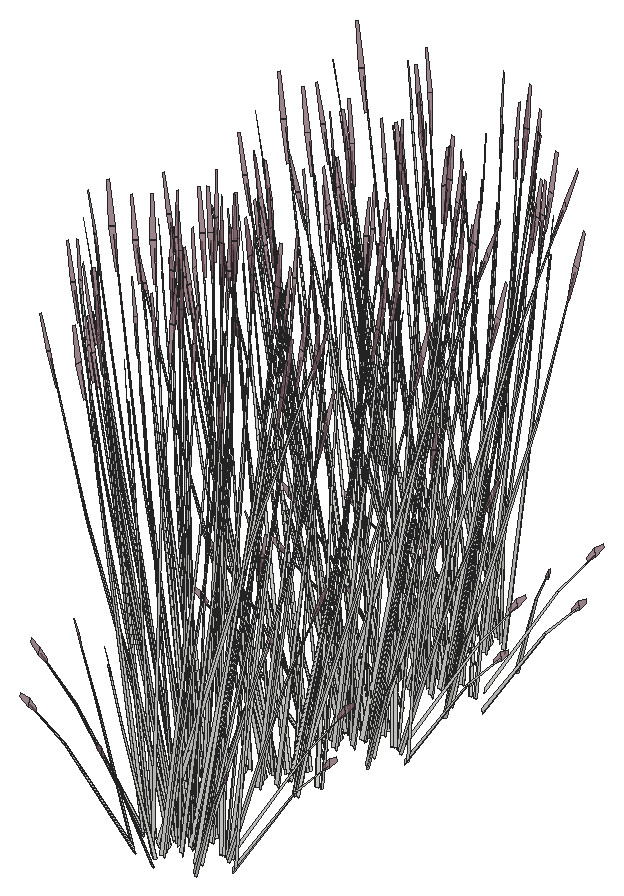
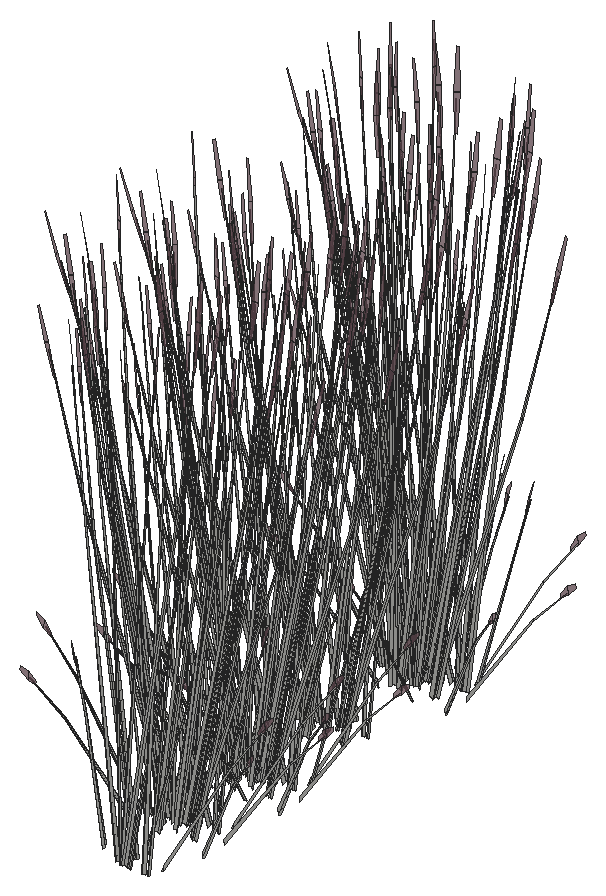
# SketchUp Ruby script. Lengths in inches.
U = 1.inch
M = Sketchup.active_model
def pt(a) = Geom::Point3d.new(a.map { |v| v * U })
def face(e, loops, mat)
  f = e.add_face(loops[0].map { |a| pt(a) })
  loops[1..].each { |l| e.add_face(l.map { |a| pt(a) }).erase! }
  f.material = f.back_material = mat if mat
  f
end
# faces: each face lists its corners as indices into pts; further lists are holes
def faces(e, pts, list, mat = nil) = list.each { |f| face(e, (f[0].is_a?(Array) ? f : [f]).map { |l| l.map { |i| pts[i] } }, mat) }
# xy, xz, yz: faces in a plane at the given z, y or x. An outline is a flat list of corners, or four numbers for a rectangle; further outlines are holes
def ring(l) = l.size == 4 ? [[l[0], l[1]], [l[2], l[1]], [l[2], l[3]], [l[0], l[3]]] : l.each_slice(2).to_a
def flat(e, list, mat, &to3) = list.each { |f| face(e, (f[0].is_a?(Array) ? f : [f]).map { |l| ring(l).map { |u, v| to3.(u, v) } }, mat) }
def xy(e, z, list, mat = nil) = flat(e, list, mat) { |x, y| [x, y, z] }
def xz(e, y, list, mat = nil) = flat(e, list, mat) { |x, z| [x, y, z] }
def yz(e, x, list, mat = nil) = flat(e, list, mat) { |y, z| [x, y, z] }
def lines(e, pts, list) = list.each { |a, b| e.add_line(pt(pts[a]), pt(pts[b])) }
# prism: a flat outline (further loops are holes) pulled along v
def prism(e, loops, v, mat = nil)
  f = face(e, loops, mat); d = Geom::Vector3d.new(v.map { |x| x * U })
  f.pushpull(f.normal.samedirection?(d) ? d.length : -d.length)
end
def box(e, o, s, mat = nil) = prism(e, [[o, [o[0] + s[0], o[1], o[2]], [o[0] + s[0], o[1] + s[1], o[2]], [o[0], o[1] + s[1], o[2]]]], [0, 0, s[2]], mat)
def at(x, y, z, deg = 0) = Geom::Transformation.translation(pt([x, y, z])) * Geom::Transformation.rotation(ORIGIN, Z_AXIS, deg.degrees)
def axes(o, x, y, z) = Geom::Transformation.new([*x, 0, *y, 0, *z, 0, *pt(o).to_a, 1])
def part(name) = M.definitions.add(name)
# library, detail: a bought-in or finely detailed component or shape, given as its bounding box
def library(name, o, s) = part(name).tap { |d| box(d.entities, o, s) }
def detail(e, o, s) = box(e.add_group.entities, o, s)
def put(e, d, t, mat = nil) = e.add_instance(d, t).tap { |i| i.material = mat if mat }
def group(e, t, mat = nil) = e.add_group.tap { |g| g.transformation = t; g.material = mat if mat }.entities
root = M.entities
M.materials.add("LightPink_Translucent").color = [144, 107, 117]
M.materials["LightPink_Translucent"].alpha = 0.75
c1 = part("blade")
p = [[2.15,0.21,22],[0,0.17,0],[0.09,0.45,0],[2.18,0.31,22],[2.29,0.31,22],[0.38,0.45,0],
  [2.48,0.24,33],[2.49,0.24,33],[2.48,0.22,33]]
faces(c1.entities,p,[[0,1,2,3],[4,5,2,3],[6,3,4,7],[8,0,3,6]])
c2 = part("seeds")
p = [[0.3,-0.1,1.38],[-0.01,-0.03,1.59],[-0.01,-0.03,0.03],[0.14,-0.07,-0.07],[0.29,-0.03,3],[0.15,0.01,3.11]]
faces(c2.entities,p,[[0,1,2,3],[1,0,4,5]],"LightPink_Translucent")
c3 = part("blade with seeds")
put(c3.entities,c1,at(0,0,0))
put(c3.entities,c2,axes([2.4,0.25,30.99],[1.5799,-0.05474,1.17369],[-0.12525,1.92788,0.29478],[-0.07173,-0.02425,1.56792]))
put(root,c3,axes([272.2,320.66,123.6],[-0.15005,0.02351,1.76342],[-0.82981,-0.26461,-0.26939],[0.01392,-0.22072,0.30037]))
put(root,c3,axes([269.52,321.47,123.6],[-0.08666,0.08595,1.76342],[-0.87574,0.18531,-0.26939],[-0.21156,-0.16858,0.30037]))
put(root,c3,axes([270.97,323.83,124.2],[-0.36739,-0.66907,-0.69835],[1.05831,-0.24096,-0.18329],[-0.04061,-0.22656,1.54149]))
put(root,c3,axes([275.88,321.79,123.6],[-0.1339,-0.0514,1.76342],[-0.34394,-0.57425,-0.26939],[0.23202,-0.15583,0.30037]))
put(root,c3,axes([270.82,321.91,124.48],[-0.55932,-0.6538,0],[0.93577,-0.36461,-0.51607],[0.21313,-0.08304,1.63711]))
put(root,c3,axes([272.05,321.12,124.23],[-0.61821,0.37431,-0.03893],[-0.56645,-0.40995,-0.17649],[-0.03988,-0.11616,0.58215]))
put(root,c3,axes([268.8,323.74,124.125],[0,-0.65246,-0.49651],[1.00089,0,0],[0,-0.1486,1.57504]))
put(root,c3,axes([271.58,321.81,124.125],[0.83726,-0.32623,-0.49651],[0.50045,0.58498,0],[0.19069,-0.0743,1.57504]))
put(root,c3,axes([272.57,323.15,124.17],[0.60257,-0.49041,-0.62353],[0.74854,0.44469,-0.16365],[0.24146,-0.12234,1.37633]))
put(root,c3,axes([271.53,324.01,124.32],[0.43405,-0.58792,-0.44739],[0.90188,0.28295,0.21531],[0,-0.13553,1.43643]))
put(root,c3,axes([271.92,323.72,124.77],[-0.10425,-0.7445,-0.29095],[1.08575,-0.04502,-0.50002],[0.19119,-0.09917,1.59708]))
put(root,c3,axes([269.23,323.75,124.14],[0.62448,-0.40708,-0.30978],[0.62448,0.40708,0.30978],[0,-0.13112,1.38974]))
put(root,c3,axes([268.98,321.8,124.23],[-0.25807,0.53277,-0.03893],[-0.79428,-0.16389,-0.17649],[-0.1206,-0.08714,0.58215]))
put(root,c3,axes([271.42,324.5,124.77],[-1.00749,-0.31132,-0.29095],[0.48511,-0.65709,-0.50002],[-0.03166,-0.16133,1.59708]))
put(root,c3,axes([268.55,324.23,124.48],[-1.11865,0,0],[0,-0.72922,-0.51607],[0,-0.16609,1.63711]))
put(root,c3,axes([271.78,322.07,124.14],[0.83462,0.16144,-0.30978],[-0.21015,0.56852,0.30978],[0.16826,-0.06556,1.38974]))
put(root,c3,axes([269.42,324.04,124.4375],[-0.83213,0.54855,0.30756],[-0.83263,-0.54278,-0.36492],[-0.02906,-0.15578,1.64885]))
put(root,c3,axes([271.67,325.1875,124.55],[0.23711,-0.77313,-0.23429],[1.12425,0.13477,0.51271],[-0.19645,-0.10677,1.5644]))
put(root,c3,axes([274.94,322.07,124.48],[0.55932,-0.6538,0],[0.93577,0.36461,-0.51607],[0.21313,0.08304,1.63711]))
put(root,c3,axes([271.59,324.87,124.32],[-0.53742,-0.54764,-0.44739],[0.81403,-0.38564,0.21531],[-0.17391,-0.06776,1.43643]))
put(root,c3,axes([277.14,324.66,124.09],[-0.57619,0.0783,1.41583],[-0.09171,-0.62326,0.08104],[0.40356,-0.09434,0.80566]))
put(root,c3,axes([278.19,324.11,124.37],[-0.55463,-0.41721,-0.06488],[0.60744,-0.38228,-0.29416],[0.17212,-0.02691,0.97024]))
put(root,c3,axes([273.1,324.16,124.3125],[0,-0.75495,0],[1.11865,0,0],[0,0,1.79456]))
put(root,c3,axes([271.11,325.08,124.17],[-0.9306,-0.10697,-0.62353],[0.19638,-0.65984,-0.16365],[-0.27771,-0.07995,1.37633]))
put(root,c3,axes([273.38,324.75,124.4],[-0.83213,-0.56158,-0.06131],[0.83263,-0.56193,0],[-0.02906,-0.01961,1.75571]))
put(root,c3,axes([270.89,323.23,123.7],[-0.88056,0.26122,1.28929],[-0.28027,-0.74951,0.50096],[0.54072,0.01247,1.46642]))
put(root,c3,axes([277.77,324.25,123.6],[-0.04675,-0.09906,1.76342],[0.32428,-0.57943,-0.26939],[0.32711,-0.00833,0.30037]))
put(root,c3,axes([268.12,324.15,123.6],[0.02269,0.10283,1.76342],[-0.45738,0.53699,-0.26939],[-0.32488,-0.02707,0.30037]))
put(root,c3,axes([270.12,326.09,124.14],[-0.21015,-0.56852,-0.30978],[0.83462,-0.16144,0.30978],[-0.16826,-0.06556,1.38974]))
put(root,c3,axes([273.17,323.62,124.77],[0.90324,-0.43318,-0.29095],[0.60064,0.61207,-0.50002],[0.22285,0.06216,1.59708]))
put(root,c3,axes([269.89,326.33,124.125],[-0.83726,-0.32623,-0.49651],[0.50045,-0.58498,0],[-0.19069,-0.0743,1.57504]))
put(root,c3,axes([275.45,322.47,124.125],[0.83726,0.32623,-0.49651],[-0.50045,0.58498,0],[0.19069,0.0743,1.57504]))
put(root,c3,axes([273.86,324.33,124.3125],[1.00089,0,0],[0,0.67548,0],[0,0,1.78407]))
put(root,c3,axes([272.17,325.18,124.77],[-0.90324,0.43318,-0.29095],[-0.60064,-0.61207,-0.50002],[-0.22285,-0.06216,1.59708]))
put(root,c3,axes([275.22,322.71,124.14],[0.21015,0.56852,-0.30978],[-0.83462,0.16144,0.30978],[0.16826,0.06556,1.38974]))
put(root,c3,axes([272.64,325.9,124.3125],[-0.29189,-0.56252,0],[0.83351,-0.19699,0],[0,0,1.54371]))
put(root,c3,axes([273.73,325.82,124.29],[0.93921,-0.22138,-0.19198],[0.33003,0.6377,0.00008],[0.10367,-0.02447,1.73897]))
put(root,c3,axes([273.84,324.62,124.32],[0.62448,0.42144,0],[-0.62448,0.42144,0],[0,0,1.69266]))
put(root,c3,axes([274.23,323.72,124.17],[0.9306,0.10697,-0.62353],[-0.19638,0.65984,-0.16365],[0.27771,0.07995,1.37633]))
put(root,c3,axes([272.43,326.16,124.3],[-0.90188,-0.29293,0],[0.43405,-0.60866,0],[0,0,1.62707]))
put(root,c3,axes([273.18,325.38,124.57],[-0.87356,-0.52515,-0.25192],[0.73507,-0.5897,0.5513],[-0.23523,0.06143,1.68216]))
put(root,c3,axes([273.67,324.46,124.4],[0,0.75458,-0.05637],[-1.11865,0,0],[0,0.02371,1.79368]))
put(root,c3,axes([273.75,323.93,124.32],[0.53742,0.54764,-0.44739],[-0.81403,0.38564,0.21531],[0.17391,0.06776,1.43643]))
put(root,c3,axes([270.4,326.72,124.48],[-0.55932,0.6538,0],[-0.93577,-0.36461,-0.51607],[-0.21313,-0.08304,1.63711]))
put(root,c3,axes([272.74,325.27,124.32],[-0.97146,0.04028,-0.44739],[-0.08785,-0.66859,0.21531],[-0.17391,0.06776,1.43643]))
put(root,c3,axes([273.45,326.17,124.3125],[0.90188,0.29293,0],[-0.43405,0.60866,0],[0,0,1.74954]))
put(root,c3,axes([273.8125,326.82,124.3],[-0.55235,-0.65609,-0.05142],[0.93577,-0.36461,0.51607],[-0.23059,0.06247,1.6363]))
put(root,c3,axes([273.13,325.92,124.4],[0.38895,0.74956,-0.06012],[-1.11135,0.26265,0],[0.01358,0.02618,1.72173]))
put(root,c3,axes([273.5625,326.73,124.14],[-0.83462,-0.16144,-0.30978],[0.21015,-0.56852,0.30978],[-0.16826,0.06556,1.38974]))
put(root,c3,axes([276.79,324.56,124.48],[1.11865,0,0],[0,0.72922,-0.51607],[0,0.16609,1.63711]))
put(root,c3,axes([276.34,324.9375,124.31],[-1.1181,-0.00522,-0.04976],[0,-0.72922,0.49943],[-0.03514,0.166,1.58352]))
put(root,c3,axes([273.92,324.3,124.77],[1.00749,0.31132,-0.29095],[-0.48511,0.65709,-0.50002],[0.03166,0.16133,1.59708]))
put(root,c3,axes([276.11,325.05,124.14],[-0.62448,0.40708,-0.30978],[-0.62448,-0.40708,0.30978],[0,0.13112,1.38974]))
put(root,c3,axes([273.42,325.08,124.77],[0.10425,0.7445,-0.29095],[-1.08575,0.04502,-0.50002],[-0.19119,0.09917,1.59708]))
put(root,c3,axes([273.81,324.79,124.32],[-0.43405,0.58792,-0.44739],[-0.90188,-0.28295,0.21531],[0,0.13553,1.43643]))
put(root,c3,axes([272.77,325.65,124.17],[-0.60257,0.49041,-0.62353],[-0.74854,-0.44469,-0.16365],[-0.24146,0.12234,1.37633]))
put(root,c3,axes([273.84,326.48,124.4375],[1.11998,0.21207,0.30756],[-0.2802,0.75803,-0.36492],[-0.18537,0.09487,1.64885]))
put(root,c3,axes([273.76,326.99,124.125],[-0.83726,0.32623,-0.49651],[-0.50045,-0.58498,0],[-0.19069,0.0743,1.57504]))
put(root,c3,axes([276.54,325.06,124.125],[0,0.65246,-0.49651],[-1.00089,0,0],[0,0.1486,1.57504]))
put(root,c3,axes([274.52,326.89,124.48],[0.55932,0.6538,0],[-0.93577,0.36461,-0.51607],[-0.21313,0.08304,1.63711]))
put(root,c3,axes([275.41,327.11,123.6],[0.06518,-0.0942,1.76342],[0.82057,-0.27742,-0.26939],[0.24877,0.14358,0.30037]))
put(root,c3,axes([274.33,324.97,124.2],[0.32803,0.59738,-0.69212],[-0.94492,0.21515,-0.18165],[0.03626,0.20229,1.52773]))
put(root,c3,axes([267.875,327.03,123.6],[0.12,0.06519,1.76342],[0.20347,0.60397,-0.26939],[-0.26596,0.12879,0.30037]))
put(root,c3,axes([271.58,327.09,123.6],[0.14478,-0.0355,1.76342],[0.8709,0.19542,-0.26939],[0.02547,0.22025,0.30037]))
put(root,c3,axes([270.97,336.8125,125.11],[-0.36739,-0.66907,-0.69835],[1.05831,-0.24096,-0.18329],[-0.04061,-0.22656,1.54149]))
put(root,c3,axes([268.8,336.72,125.03],[0,-0.65246,-0.49651],[1.00089,0,0],[0,-0.1486,1.57504]))
put(root,c3,axes([271.58,334.79,125.03],[0.83726,-0.32623,-0.49651],[0.50045,0.58498,0],[0.19069,-0.0743,1.57504]))
put(root,c3,axes([272.57,336.125,125.07],[0.60257,-0.49041,-0.62353],[0.74854,0.44469,-0.16365],[0.24146,-0.12234,1.37633]))
put(root,c3,axes([271.53,336.98,125.22],[0.43405,-0.58792,-0.44739],[0.90188,0.28295,0.21531],[0,-0.13553,1.43643]))
put(root,c3,axes([269.23,336.73,125.04],[0.62448,-0.40708,-0.30978],[0.62448,0.40708,0.30978],[0,-0.13112,1.38974]))
put(root,c3,axes([271.78,335.04,125.04],[0.83462,0.16144,-0.30978],[-0.21015,0.56852,0.30978],[0.16826,-0.06556,1.38974]))
put(root,c3,axes([271.59,337.85,125.22],[-0.53742,-0.54764,-0.44739],[0.81403,-0.38564,0.21531],[-0.17391,-0.06776,1.43643]))
put(root,c3,axes([271.11,338.06,125.07],[-0.9306,-0.10697,-0.62353],[0.19638,-0.65984,-0.16365],[-0.27771,-0.07995,1.37633]))
put(root,c3,axes([270.12,339.06,125.04],[-0.21015,-0.56852,-0.30978],[0.83462,-0.16144,0.30978],[-0.16826,-0.06556,1.38974]))
put(root,c3,axes([269.89,339.31,125.03],[-0.83726,-0.32623,-0.49651],[0.50045,-0.58498,0],[-0.19069,-0.0743,1.57504]))
put(root,c3,axes([275.45,335.45,125.03],[0.83726,0.32623,-0.49651],[-0.50045,0.58498,0],[0.19069,0.0743,1.57504]))
put(root,c3,axes([275.22,335.6875,125.04],[0.21015,0.56852,-0.30978],[-0.83462,0.16144,0.30978],[0.16826,0.06556,1.38974]))
put(root,c3,axes([274.23,336.69,125.07],[0.9306,0.10697,-0.62353],[-0.19638,0.65984,-0.16365],[0.27771,0.07995,1.37633]))
put(root,c3,axes([273.75,336.9,125.22],[0.53742,0.54764,-0.44739],[-0.81403,0.38564,0.21531],[0.17391,0.06776,1.43643]))
put(root,c3,axes([272.74,338.24,125.22],[-0.97146,0.04028,-0.44739],[-0.08785,-0.66859,0.21531],[-0.17391,0.06776,1.43643]))
put(root,c3,axes([272.2,343.92,123.82],[-0.15005,0.02351,1.76342],[-0.82981,-0.26461,-0.26939],[0.01392,-0.22072,0.30037]))
put(root,c3,axes([273.5625,339.71,125.04],[-0.83462,-0.16144,-0.30978],[0.21015,-0.56852,0.30978],[-0.16826,0.06556,1.38974]))
put(root,c3,axes([276.11,338.02,125.04],[-0.62448,0.40708,-0.30978],[-0.62448,-0.40708,0.30978],[0,0.13112,1.38974]))
put(root,c3,axes([273.81,337.77,125.22],[-0.43405,0.58792,-0.44739],[-0.90188,-0.28295,0.21531],[0,0.13553,1.43643]))
put(root,c3,axes([272.77,338.63,125.07],[-0.60257,0.49041,-0.62353],[-0.74854,-0.44469,-0.16365],[-0.24146,0.12234,1.37633]))
put(root,c3,axes([273.76,339.97,125.03],[-0.83726,0.32623,-0.49651],[-0.50045,-0.58498,0],[-0.19069,0.0743,1.57504]))
put(root,c3,axes([276.54,338.04,125.03],[0,0.65246,-0.49651],[-1.00089,0,0],[0,0.1486,1.57504]))
put(root,c3,axes([269.52,344.72,123.82],[-0.08666,0.08595,1.76342],[-0.87574,0.18531,-0.26939],[-0.21156,-0.16858,0.30037]))
put(root,c3,axes([270.97,347.09,124.42],[-0.36739,-0.66907,-0.69835],[1.05831,-0.24096,-0.18329],[-0.04061,-0.22656,1.54149]))
put(root,c3,axes([275.88,345.04,123.82],[-0.1339,-0.0514,1.76342],[-0.34394,-0.57425,-0.26939],[0.23202,-0.15583,0.30037]))
put(root,c3,axes([274.33,337.95,125.11],[0.32803,0.59738,-0.69212],[-0.94492,0.21515,-0.18165],[0.03626,0.20229,1.52773]))
put(root,c3,axes([272.05,344.375,124.45],[-0.61821,0.37431,-0.03893],[-0.56645,-0.40995,-0.17649],[-0.03988,-0.11616,0.58215]))
put(root,c3,axes([268.8,346.99,124.34],[0,-0.65246,-0.49651],[1.00089,0,0],[0,-0.1486,1.57504]))
put(root,c3,axes([271.58,345.0625,124.34],[0.83726,-0.32623,-0.49651],[0.50045,0.58498,0],[0.19069,-0.0743,1.57504]))
put(root,c3,axes([272.57,346.4,124.38],[0.60257,-0.49041,-0.62353],[0.74854,0.44469,-0.16365],[0.24146,-0.12234,1.37633]))
put(root,c3,axes([271.53,347.26,124.53],[0.43405,-0.58792,-0.44739],[0.90188,0.28295,0.21531],[0,-0.13553,1.43643]))
put(root,c3,axes([271.92,346.97,124.99],[-0.10425,-0.7445,-0.29095],[1.08575,-0.04502,-0.50002],[0.19119,-0.09917,1.59708]))
put(root,c3,axes([269.23,347.01,124.35],[0.62448,-0.40708,-0.30978],[0.62448,0.40708,0.30978],[0,-0.13112,1.38974]))
put(root,c3,axes([268.98,345.06,124.45],[-0.25807,0.53277,-0.03893],[-0.79428,-0.16389,-0.17649],[-0.1206,-0.08714,0.58215]))
put(root,c3,axes([271.42,347.75,124.99],[-1.00749,-0.31132,-0.29095],[0.48511,-0.65709,-0.50002],[-0.03166,-0.16133,1.59708]))
put(root,c3,axes([271.78,345.32,124.35],[0.83462,0.16144,-0.30978],[-0.21015,0.56852,0.30978],[0.16826,-0.06556,1.38974]))
put(root,c3,axes([271.67,348.4375,124.76],[0.23711,-0.77313,-0.23429],[1.12425,0.13477,0.51271],[-0.19645,-0.10677,1.5644]))
put(root,c3,axes([271.59,348.125,124.53],[-0.53742,-0.54764,-0.44739],[0.81403,-0.38564,0.21531],[-0.17391,-0.06776,1.43643]))
put(root,c3,axes([277.14,347.91,124.31],[-0.57619,0.0783,1.41583],[-0.09171,-0.62326,0.08104],[0.40356,-0.09434,0.80566]))
put(root,c3,axes([278.19,347.36,124.58],[-0.55463,-0.41721,-0.06488],[0.60744,-0.38228,-0.29416],[0.17212,-0.02691,0.97024]))
put(root,c3,axes([271.11,348.33,124.38],[-0.9306,-0.10697,-0.62353],[0.19638,-0.65984,-0.16365],[-0.27771,-0.07995,1.37633]))
put(root,c3,axes([270.89,346.49,123.92],[-0.88056,0.26122,1.28929],[-0.28027,-0.74951,0.50096],[0.54072,0.01247,1.46642]))
put(root,c3,axes([277.77,347.5,123.82],[-0.04675,-0.09906,1.76342],[0.32428,-0.57943,-0.26939],[0.32711,-0.00833,0.30037]))
put(root,c3,axes([268.12,347.4,123.82],[0.02269,0.10283,1.76342],[-0.45738,0.53699,-0.26939],[-0.32488,-0.02707,0.30037]))
put(root,c3,axes([270.12,349.34,124.35],[-0.21015,-0.56852,-0.30978],[0.83462,-0.16144,0.30978],[-0.16826,-0.06556,1.38974]))
put(root,c3,axes([273.17,346.87,124.99],[0.90324,-0.43318,-0.29095],[0.60064,0.61207,-0.50002],[0.22285,0.06216,1.59708]))
put(root,c3,axes([269.89,349.58,124.34],[-0.83726,-0.32623,-0.49651],[0.50045,-0.58498,0],[-0.19069,-0.0743,1.57504]))
put(root,c3,axes([275.45,345.72,124.34],[0.83726,0.32623,-0.49651],[-0.50045,0.58498,0],[0.19069,0.0743,1.57504]))
put(root,c3,axes([272.17,348.43,124.99],[-0.90324,0.43318,-0.29095],[-0.60064,-0.61207,-0.50002],[-0.22285,-0.06216,1.59708]))
put(root,c3,axes([275.22,345.96,124.35],[0.21015,0.56852,-0.30978],[-0.83462,0.16144,0.30978],[0.16826,0.06556,1.38974]))
put(root,c3,axes([273.73,349.08,124.51],[0.93921,-0.22138,-0.19198],[0.33003,0.6377,0.00008],[0.10367,-0.02447,1.73897]))
put(root,c3,axes([274.23,346.97,124.38],[0.9306,0.10697,-0.62353],[-0.19638,0.65984,-0.16365],[0.27771,0.07995,1.37633]))
put(root,c3,axes([273.18,348.63,124.79],[-0.87356,-0.52515,-0.25192],[0.73507,-0.5897,0.5513],[-0.23523,0.06143,1.68216]))
put(root,c3,axes([273.75,347.18,124.53],[0.53742,0.54764,-0.44739],[-0.81403,0.38564,0.21531],[0.17391,0.06776,1.43643]))
put(root,c3,axes([272.74,348.52,124.53],[-0.97146,0.04028,-0.44739],[-0.08785,-0.66859,0.21531],[-0.17391,0.06776,1.43643]))
put(root,c3,axes([273.8125,350.07,124.52],[-0.55235,-0.65609,-0.05142],[0.93577,-0.36461,0.51607],[-0.23059,0.06247,1.6363]))
put(root,c3,axes([272.2,354.45,124.14],[-0.15005,0.02351,1.76342],[-0.82981,-0.26461,-0.26939],[0.01392,-0.22072,0.30037]))
put(root,c3,axes([273.5625,349.99,124.35],[-0.83462,-0.16144,-0.30978],[0.21015,-0.56852,0.30978],[-0.16826,0.06556,1.38974]))
put(root,c3,axes([276.34,348.19,124.52],[-1.1181,-0.00522,-0.04976],[0,-0.72922,0.49943],[-0.03514,0.166,1.58352]))
put(root,c3,axes([273.92,347.56,124.99],[1.00749,0.31132,-0.29095],[-0.48511,0.65709,-0.50002],[0.03166,0.16133,1.59708]))
put(root,c3,axes([276.11,348.3,124.35],[-0.62448,0.40708,-0.30978],[-0.62448,-0.40708,0.30978],[0,0.13112,1.38974]))
put(root,c3,axes([273.42,348.34,124.99],[0.10425,0.7445,-0.29095],[-1.08575,0.04502,-0.50002],[-0.19119,0.09917,1.59708]))
put(root,c3,axes([273.81,348.05,124.53],[-0.43405,0.58792,-0.44739],[-0.90188,-0.28295,0.21531],[0,0.13553,1.43643]))
put(root,c3,axes([272.77,348.91,124.38],[-0.60257,0.49041,-0.62353],[-0.74854,-0.44469,-0.16365],[-0.24146,0.12234,1.37633]))
put(root,c3,axes([273.76,350.24,124.34],[-0.83726,0.32623,-0.49651],[-0.50045,-0.58498,0],[-0.19069,0.0743,1.57504]))
put(root,c3,axes([276.54,348.3125,124.34],[0,0.65246,-0.49651],[-1.00089,0,0],[0,0.1486,1.57504]))
put(root,c3,axes([269.52,355.26,124.14],[-0.08666,0.08595,1.76342],[-0.87574,0.18531,-0.26939],[-0.21156,-0.16858,0.30037]))
put(root,c3,axes([270.97,357.62,124.74],[-0.36739,-0.66907,-0.69835],[1.05831,-0.24096,-0.18329],[-0.04061,-0.22656,1.54149]))
put(root,c3,axes([275.88,355.58,124.14],[-0.1339,-0.0514,1.76342],[-0.34394,-0.57425,-0.26939],[0.23202,-0.15583,0.30037]))
put(root,c3,axes([275.41,350.36,123.82],[0.06518,-0.0942,1.76342],[0.82057,-0.27742,-0.26939],[0.24877,0.14358,0.30037]))
put(root,c3,axes([274.33,348.22,124.42],[0.32803,0.59738,-0.69212],[-0.94492,0.21515,-0.18165],[0.03626,0.20229,1.52773]))
put(root,c3,axes([267.875,350.28,123.82],[0.12,0.06519,1.76342],[0.20347,0.60397,-0.26939],[-0.26596,0.12879,0.30037]))
put(root,c3,axes([268.8,357.53,124.66],[0,-0.65246,-0.49651],[1.00089,0,0],[0,-0.1486,1.57504]))
put(root,c3,axes([271.58,355.6,124.66],[0.83726,-0.32623,-0.49651],[0.50045,0.58498,0],[0.19069,-0.0743,1.57504]))
put(root,c3,axes([272.57,356.93,124.7],[0.60257,-0.49041,-0.62353],[0.74854,0.44469,-0.16365],[0.24146,-0.12234,1.37633]))
put(root,c3,axes([271.58,350.34,123.82],[0.14478,-0.0355,1.76342],[0.8709,0.19542,-0.26939],[0.02547,0.22025,0.30037]))
put(root,c3,axes([271.53,357.79,124.86],[0.43405,-0.58792,-0.44739],[0.90188,0.28295,0.21531],[0,-0.13553,1.43643]))
put(root,c3,axes([271.92,357.5,125.3125],[-0.10425,-0.7445,-0.29095],[1.08575,-0.04502,-0.50002],[0.19119,-0.09917,1.59708]))
put(root,c3,axes([269.23,357.54,124.67],[0.62448,-0.40708,-0.30978],[0.62448,0.40708,0.30978],[0,-0.13112,1.38974]))
put(root,c3,axes([271.42,358.28,125.3125],[-1.00749,-0.31132,-0.29095],[0.48511,-0.65709,-0.50002],[-0.03166,-0.16133,1.59708]))
put(root,c3,axes([271.78,355.85,124.67],[0.83462,0.16144,-0.30978],[-0.21015,0.56852,0.30978],[0.16826,-0.06556,1.38974]))
put(root,c3,axes([271.59,358.66,124.86],[-0.53742,-0.54764,-0.44739],[0.81403,-0.38564,0.21531],[-0.17391,-0.06776,1.43643]))
put(root,c3,axes([271.11,358.87,124.7],[-0.9306,-0.10697,-0.62353],[0.19638,-0.65984,-0.16365],[-0.27771,-0.07995,1.37633]))
put(root,c3,axes([270.89,357.02,124.24],[-0.88056,0.26122,1.28929],[-0.28027,-0.74951,0.50096],[0.54072,0.01247,1.46642]))
put(root,c3,axes([277.77,358.04,124.14],[-0.04675,-0.09906,1.76342],[0.32428,-0.57943,-0.26939],[0.32711,-0.00833,0.30037]))
put(root,c3,axes([268.12,357.9375,124.14],[0.02269,0.10283,1.76342],[-0.45738,0.53699,-0.26939],[-0.32488,-0.02707,0.30037]))
put(root,c3,axes([270.12,359.875,124.67],[-0.21015,-0.56852,-0.30978],[0.83462,-0.16144,0.30978],[-0.16826,-0.06556,1.38974]))
put(root,c3,axes([273.17,357.41,125.3125],[0.90324,-0.43318,-0.29095],[0.60064,0.61207,-0.50002],[0.22285,0.06216,1.59708]))
put(root,c3,axes([269.89,360.12,124.66],[-0.83726,-0.32623,-0.49651],[0.50045,-0.58498,0],[-0.19069,-0.0743,1.57504]))
put(root,c3,axes([275.45,356.26,124.66],[0.83726,0.32623,-0.49651],[-0.50045,0.58498,0],[0.19069,0.0743,1.57504]))
put(root,c3,axes([272.17,358.97,125.3125],[-0.90324,0.43318,-0.29095],[-0.60064,-0.61207,-0.50002],[-0.22285,-0.06216,1.59708]))
put(root,c3,axes([275.22,356.5,124.67],[0.21015,0.56852,-0.30978],[-0.83462,0.16144,0.30978],[0.16826,0.06556,1.38974]))
put(root,c3,axes([273.73,359.61,124.83],[0.93921,-0.22138,-0.19198],[0.33003,0.6377,0.00008],[0.10367,-0.02447,1.73897]))
put(root,c3,axes([274.23,357.51,124.7],[0.9306,0.10697,-0.62353],[-0.19638,0.65984,-0.16365],[0.27771,0.07995,1.37633]))
put(root,c3,axes([273.18,359.16,125.11],[-0.87356,-0.52515,-0.25192],[0.73507,-0.5897,0.5513],[-0.23523,0.06143,1.68216]))
put(root,c3,axes([273.75,357.72,124.86],[0.53742,0.54764,-0.44739],[-0.81403,0.38564,0.21531],[0.17391,0.06776,1.43643]))
put(root,c3,axes([272.74,359.05,124.86],[-0.97146,0.04028,-0.44739],[-0.08785,-0.66859,0.21531],[-0.17391,0.06776,1.43643]))
put(root,c3,axes([272.2,364.27,124.17],[-0.15005,0.02351,1.76342],[-0.82981,-0.26461,-0.26939],[0.01392,-0.22072,0.30037]))
put(root,c3,axes([273.5625,360.52,124.67],[-0.83462,-0.16144,-0.30978],[0.21015,-0.56852,0.30978],[-0.16826,0.06556,1.38974]))
put(root,c3,axes([273.92,358.09,125.3125],[1.00749,0.31132,-0.29095],[-0.48511,0.65709,-0.50002],[0.03166,0.16133,1.59708]))
put(root,c3,axes([276.11,358.83,124.67],[-0.62448,0.40708,-0.30978],[-0.62448,-0.40708,0.30978],[0,0.13112,1.38974]))
put(root,c3,axes([273.42,358.87,125.3125],[0.10425,0.7445,-0.29095],[-1.08575,0.04502,-0.50002],[-0.19119,0.09917,1.59708]))
put(root,c3,axes([273.81,358.58,124.86],[-0.43405,0.58792,-0.44739],[-0.90188,-0.28295,0.21531],[0,0.13553,1.43643]))
put(root,c3,axes([269.52,365.08,124.17],[-0.08666,0.08595,1.76342],[-0.87574,0.18531,-0.26939],[-0.21156,-0.16858,0.30037]))
put(root,c3,axes([272.77,359.44,124.7],[-0.60257,0.49041,-0.62353],[-0.74854,-0.44469,-0.16365],[-0.24146,0.12234,1.37633]))
put(root,c3,axes([270.97,367.44,124.77],[-0.36739,-0.66907,-0.69835],[1.05831,-0.24096,-0.18329],[-0.04061,-0.22656,1.54149]))
put(root,c3,axes([275.88,365.4,124.17],[-0.1339,-0.0514,1.76342],[-0.34394,-0.57425,-0.26939],[0.23202,-0.15583,0.30037]))
put(root,c3,axes([273.76,360.78,124.66],[-0.83726,0.32623,-0.49651],[-0.50045,-0.58498,0],[-0.19069,0.0743,1.57504]))
put(root,c3,axes([276.54,358.85,124.66],[0,0.65246,-0.49651],[-1.00089,0,0],[0,0.1486,1.57504]))
put(root,c3,axes([275.41,360.9,124.14],[0.06518,-0.0942,1.76342],[0.82057,-0.27742,-0.26939],[0.24877,0.14358,0.30037]))
put(root,c3,axes([274.33,358.76,124.74],[0.32803,0.59738,-0.69212],[-0.94492,0.21515,-0.18165],[0.03626,0.20229,1.52773]))
put(root,c3,axes([267.875,360.82,124.14],[0.12,0.06519,1.76342],[0.20347,0.60397,-0.26939],[-0.26596,0.12879,0.30037]))
put(root,c3,axes([268.8,367.35,124.69],[0,-0.65246,-0.49651],[1.00089,0,0],[0,-0.1486,1.57504]))
put(root,c3,axes([271.58,365.42,124.69],[0.83726,-0.32623,-0.49651],[0.50045,0.58498,0],[0.19069,-0.0743,1.57504]))
put(root,c3,axes([272.57,366.76,124.73],[0.60257,-0.49041,-0.62353],[0.74854,0.44469,-0.16365],[0.24146,-0.12234,1.37633]))
put(root,c3,axes([271.53,367.62,124.89],[0.43405,-0.58792,-0.44739],[0.90188,0.28295,0.21531],[0,-0.13553,1.43643]))
put(root,c3,axes([271.92,367.32,125.34],[-0.10425,-0.7445,-0.29095],[1.08575,-0.04502,-0.50002],[0.19119,-0.09917,1.59708]))
put(root,c3,axes([269.23,367.36,124.7],[0.62448,-0.40708,-0.30978],[0.62448,0.40708,0.30978],[0,-0.13112,1.38974]))
put(root,c3,axes([271.42,368.1,125.34],[-1.00749,-0.31132,-0.29095],[0.48511,-0.65709,-0.50002],[-0.03166,-0.16133,1.59708]))
put(root,c3,axes([271.78,365.68,124.7],[0.83462,0.16144,-0.30978],[-0.21015,0.56852,0.30978],[0.16826,-0.06556,1.38974]))
